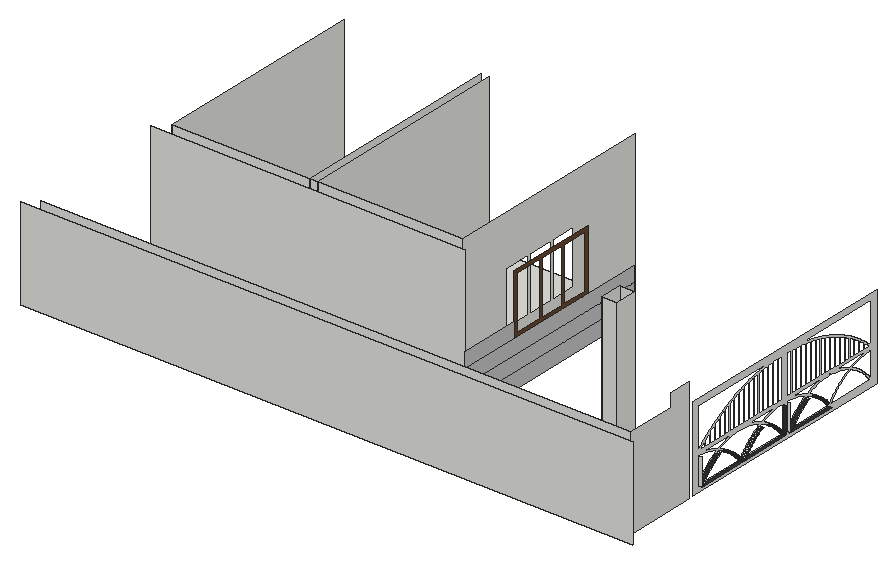
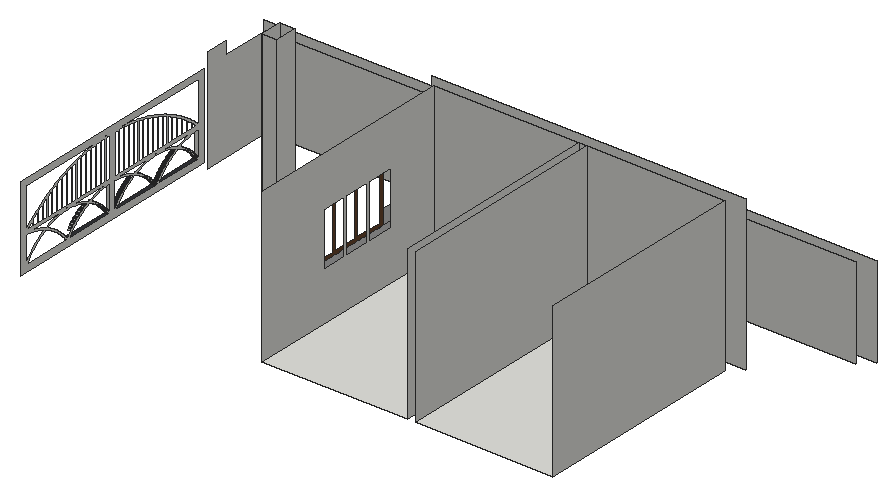
# SketchUp Ruby script. Lengths in inches.
U = 1.inch
M = Sketchup.active_model
def pt(a) = Geom::Point3d.new(a.map { |v| v * U })
def face(e, loops, mat)
  f = e.add_face(loops[0].map { |a| pt(a) })
  loops[1..].each { |l| e.add_face(l.map { |a| pt(a) }).erase! }
  f.material = f.back_material = mat if mat
  f
end
# faces: each face lists its corners as indices into pts; further lists are holes
def faces(e, pts, list, mat = nil) = list.each { |f| face(e, (f[0].is_a?(Array) ? f : [f]).map { |l| l.map { |i| pts[i] } }, mat) }
# xy, xz, yz: faces in a plane at the given z, y or x. An outline is a flat list of corners, or four numbers for a rectangle; further outlines are holes
def ring(l) = l.size == 4 ? [[l[0], l[1]], [l[2], l[1]], [l[2], l[3]], [l[0], l[3]]] : l.each_slice(2).to_a
def flat(e, list, mat, &to3) = list.each { |f| face(e, (f[0].is_a?(Array) ? f : [f]).map { |l| ring(l).map { |u, v| to3.(u, v) } }, mat) }
def xy(e, z, list, mat = nil) = flat(e, list, mat) { |x, y| [x, y, z] }
def xz(e, y, list, mat = nil) = flat(e, list, mat) { |x, z| [x, y, z] }
def yz(e, x, list, mat = nil) = flat(e, list, mat) { |y, z| [x, y, z] }
def lines(e, pts, list) = list.each { |a, b| e.add_line(pt(pts[a]), pt(pts[b])) }
# prism: a flat outline (further loops are holes) pulled along v
def prism(e, loops, v, mat = nil)
  f = face(e, loops, mat); d = Geom::Vector3d.new(v.map { |x| x * U })
  f.pushpull(f.normal.samedirection?(d) ? d.length : -d.length)
end
def box(e, o, s, mat = nil) = prism(e, [[o, [o[0] + s[0], o[1], o[2]], [o[0] + s[0], o[1] + s[1], o[2]], [o[0], o[1] + s[1], o[2]]]], [0, 0, s[2]], mat)
def at(x, y, z, deg = 0) = Geom::Transformation.translation(pt([x, y, z])) * Geom::Transformation.rotation(ORIGIN, Z_AXIS, deg.degrees)
def axes(o, x, y, z) = Geom::Transformation.new([*x, 0, *y, 0, *z, 0, *pt(o).to_a, 1])
def part(name) = M.definitions.add(name)
# library, detail: a bought-in or finely detailed component or shape, given as its bounding box
def library(name, o, s) = part(name).tap { |d| box(d.entities, o, s) }
def detail(e, o, s) = box(e.add_group.entities, o, s)
def put(e, d, t, mat = nil) = e.add_instance(d, t).tap { |i| i.material = mat if mat }
def group(e, t, mat = nil) = e.add_group.tap { |g| g.transformation = t; g.material = mat if mat }.entities
root = M.entities
M.materials.add("M02_Ash_Whisper").color = [196, 196, 196]
M.materials.add("ThomThom - Buttons1").color = [48, 49, 53]
M.materials.add("Wood_Veneer_15_1K").color = [103, 69, 45]
xy(root,24,[[66,66,174,234],[180,66,294,234]])
xy(root,32,[[474,72.225,477,111.313],[474,113.367,477,152.836],[474,159.225,477,198.633]],"ThomThom - Buttons1")
xz(root,0,[[0,24,480,96]])
xz(root,9,[[9,24,471,96]])
xz(root,57,[[57,24,303,144]])
xz(root,63,[[405,24,417,144]])
xz(root,66,[[66,24,174,144],[174,24,180,144],[180,24,294,144]])
xz(root,71,[[474,32,477,53.015]])
xz(root,81,[[405,24,417,144]])
xz(root,154,[[474,32,477,53.014]],"ThomThom - Buttons1")
xz(root,158,[[474,32,477,53.014]])
yz(root,66,[[66,24,234,144]])
yz(root,174,[[66,24,234,144]])
yz(root,180,[[66,24,234,144]])
yz(root,294,[[[66,24,234,144],[108,63,130,105],[132.007,62.883,152,105],[154.007,62.883,174,105]]])
yz(root,303,[[57,24,222,36],[57,36,222,48],[57,48,222,60],[57,60,105,72]],"M02_Ash_Whisper")
yz(root,303,[[[105,60,177,108],[132.007,62.883,132.007,104.883,130,105,130,63,108,63,108,105,130,105,132.007,104.883,152,105,154.007,104.883,174,105,174,63,154.007,62.883,154.007,104.883,152,105,152,63]]],"Wood_Veneer_15_1K")
yz(root,405,[[63,24,81,144]])
yz(root,417,[[63,24,81,144]])
yz(root,471,[[9,24,9,96,48,96,48,106,66,106,66,24]])
yz(root,474,[[[66,27,246,93],[241,56,241,88,161.003,88,161.646,87.994,163.468,87.949,165.29,87.877,167.11,87.776,168.929,87.648,170.745,87.493,172.559,87.309,174.37,87.098,176.177,86.859,177.98,86.593,179.779,86.299,181.574,85.977,183.363,85.629,185.147,85.253,186.925,84.85,188.696,84.42,190.461,83.962,192.219,83.478,193.969,82.967,195.711,82.43,197.444,81.866,199.169,81.275,200.885,80.659,202.59,80.016,204.286,79.347,205.972,78.653,207.647,77.932,209.31,77.187,210.962,76.416,212.602,75.62,214.23,74.799,215.845,73.953,217.446,73.082,219.035,72.1875,220.609,71.269,222.17,70.326,223.715,69.36,225.246,68.37,226.762,67.356,228.262,66.32,229.745,65.261,231.213,64.18,232.664,63.076,234.098,61.95,235.514,60.802,236.913,59.633,238.294,58.443,239.656,57.232],[71,56,72.344,57.232,73.588,58.338,73.706,58.443,75.087,59.633,76.486,60.802,77.902,61.95,78.318,62.277,79.336,63.076,80.787,64.18,82.255,65.261,83.048,65.828,83.738,66.32,85.238,67.356,86.754,68.37,87.778,69.032,88.285,69.36,89.83,70.326,91.391,71.269,92.509,71.921,92.965,72.1875,94.554,73.082,96.155,73.953,97.239,74.52,97.77,74.799,99.398,75.62,101.038,76.416,101.969,76.85,102.69,77.187,104.353,77.932,106.028,78.653,106.699,78.929,107.714,79.347,109.41,80.016,111.115,80.659,111.429,80.771,112.831,81.275,114.556,81.866,116.159,82.388,116.289,82.43,118.031,82.967,119.781,83.478,120.889,83.783,121.539,83.962,123.304,84.42,125.075,84.85,125.619,84.973,126.853,85.253,128.637,85.629,130.349,85.962,130.426,85.977,132.221,86.299,134.02,86.593,135.08,86.749,135.823,86.859,137.63,87.098,139.441,87.309,141.255,87.493,143.071,87.648,144.89,87.776,146.71,87.877,148.532,87.949,150.354,87.994,150.997,88,71,88],[199.66,32.254,200.052,32.779,200.649,33.547,201.259,34.304,201.883,35.05,202.52,35.784,203.171,36.507,203.834,37.218,204.51,37.918,205.198,38.604,205.899,39.279,206.612,39.94,207.336,40.589,208.072,41.225,208.819,41.847,209.578,42.455,210.347,43.05,211.127,43.631,211.917,44.198,212.718,44.751,213.528,45.288,214.347,45.812,215.176,46.32,216.014,46.814,216.861,47.292,217.716,47.755,218.58,48.202,219.451,48.634,219.589,48.7,218.181,49.31,216.395,50.004,214.583,50.628,212.748,51.18,210.893,51.661,209.021,52.069,207.134,52.403,205.236,52.664,203.329,52.85,201.416,52.962,199.5,53,197.584,52.962,195.671,52.85,193.764,52.664,191.866,52.403,189.979,52.069,188.107,51.661,186.252,51.18,184.417,50.628,182.605,50.004,180.819,49.31,179.578,48.772,179.731,48.7,179.869,48.634,180.74,48.202,181.604,47.755,182.459,47.292,183.306,46.814,184.144,46.32,184.973,45.812,185.792,45.288,186.602,44.751,187.403,44.198,188.193,43.631,188.973,43.05,189.742,42.455,190.501,41.847,191.248,41.225,191.984,40.589,192.708,39.94,193.421,39.279,194.122,38.604,194.81,37.918,195.486,37.218,196.149,36.507,196.8,35.784,197.437,35.05,198.061,34.304,198.671,33.547,199.268,32.779],[112.34,32.254,112.732,32.779,113.329,33.547,113.939,34.304,114.563,35.05,115.2,35.784,115.851,36.507,116.514,37.218,117.19,37.918,117.878,38.604,118.579,39.279,119.292,39.94,120.016,40.589,120.752,41.225,121.499,41.847,122.258,42.455,123.027,43.05,123.807,43.631,124.597,44.198,125.398,44.751,126.208,45.288,127.027,45.812,127.856,46.32,128.694,46.814,129.541,47.292,130.396,47.755,131.26,48.202,132.131,48.634,132.269,48.7,132.422,48.772,131.181,49.31,129.395,50.004,127.583,50.628,125.748,51.18,123.893,51.661,122.021,52.069,120.134,52.403,118.236,52.664,116.329,52.85,114.416,52.962,112.5,53,110.584,52.962,108.671,52.85,106.764,52.664,104.866,52.403,102.979,52.069,101.107,51.661,99.252,51.18,97.417,50.628,95.605,50.004,93.819,49.31,92.411,48.7,92.549,48.634,93.42,48.202,94.284,47.755,95.139,47.292,95.986,46.814,96.824,46.32,97.653,45.812,98.472,45.288,99.282,44.751,100.083,44.198,100.873,43.631,101.653,43.05,102.422,42.455,103.181,41.847,103.928,41.225,104.664,40.589,105.388,39.94,106.101,39.279,106.802,38.604,107.49,37.918,108.166,37.218,108.829,36.507,109.48,35.784,110.117,35.05,110.741,34.304,111.351,33.547,111.948,32.779],[113.367,32,152.836,32,152.066,33.003,150.9,34.524,149.675,35.997,148.394,37.422,147.058,38.796,145.669,40.117,144.231,41.382,142.744,42.591,141.21,43.741,139.634,44.83,138.016,45.856,136.359,46.819,134.666,47.717,133.583,48.238,131.712,47.31,130.864,46.871,130.025,46.417,129.194,45.947,128.371,45.463,127.558,44.964,126.753,44.45,125.958,43.922,125.173,43.38,124.397,42.824,123.632,42.254,122.877,41.67,122.132,41.073,121.399,40.462,120.676,39.838,119.965,39.201,119.266,38.552,118.578,37.89,117.903,37.216,117.239,36.53,116.588,35.832,115.95,35.122,115.325,34.401,114.712,33.669],[159.225,32,198.633,32,197.288,33.669,196.675,34.401,196.05,35.122,195.412,35.832,194.761,36.53,194.097,37.216,193.422,37.89,192.734,38.552,192.035,39.201,191.324,39.838,190.601,40.462,189.868,41.073,189.123,41.67,188.368,42.254,187.603,42.824,186.827,43.38,186.042,43.922,185.247,44.45,184.442,44.964,183.629,45.463,182.806,45.947,181.975,46.417,181.136,46.871,180.288,47.31,178.417,48.238,177.334,47.717,175.641,46.819,173.984,45.856,172.366,44.83,170.79,43.741,169.256,42.591,167.769,41.382,166.331,40.117,164.942,38.796,163.606,37.422,162.325,35.997,161.1,34.524,159.934,33.003,159.932,33],[72.225,32,111.313,32,110.507,33,109.968,33.669,109.355,34.401,108.73,35.122,108.092,35.832,107.441,36.53,106.778,37.216,106.102,37.89,105.414,38.552,104.715,39.201,104.004,39.838,103.281,40.462,102.548,41.073,101.803,41.67,101.048,42.254,100.283,42.824,99.507,43.38,98.722,43.922,97.927,44.45,97.122,44.964,96.309,45.463,95.486,45.947,94.655,46.417,93.816,46.871,92.968,47.31,92.391,47.597,91.195,48.131,90.334,47.717,88.641,46.819,86.984,45.856,85.366,44.83,83.79,43.741,82.256,42.591,80.769,41.382,79.331,40.117,77.942,38.796,76.606,37.422,75.325,35.997,74.1,34.524,72.934,33.003],[200.687,32,239.775,32,239.066,33.003,237.9,34.524,236.675,35.997,235.394,37.422,234.058,38.796,232.669,40.117,231.231,41.382,229.744,42.591,228.21,43.741,226.634,44.83,225.016,45.856,223.359,46.819,221.666,47.717,220.805,48.131,219.609,47.597,219.032,47.31,218.184,46.871,217.345,46.417,216.514,45.947,215.691,45.463,214.878,44.964,214.073,44.45,213.278,43.922,212.493,43.38,211.717,42.824,210.952,42.254,210.197,41.67,209.452,41.073,208.719,40.462,207.996,39.838,207.285,39.201,206.586,38.552,205.898,37.89,205.222,37.216,204.559,36.53,203.908,35.832,203.27,35.122,202.645,34.401,202.032,33.669,201.493,33],[154,32,154,53.014,152.764,52.957,151.811,52.896,150.86,52.818,149.91,52.722,148.962,52.61,148.017,52.481,147.074,52.334,146.133,52.171,145.196,51.991,144.262,51.793,143.332,51.58,142.406,51.349,141.484,51.102,140.567,50.838,139.654,50.558,138.747,50.261,137.845,49.948,136.949,49.619,136.06,49.274,134.719,48.801,135.117,48.609,136.845,47.694,138.535,46.711,140.186,45.664,141.795,44.552,143.359,43.379,144.876,42.146,146.345,40.855,147.761,39.507,149.124,38.105,150.432,36.652,151.681,35.148,152.871,33.597],[158,32,159.129,33.597,160.319,35.148,161.568,36.652,162.876,38.105,164.239,39.507,165.655,40.855,167.124,42.146,168.641,43.379,170.205,44.552,171.814,45.664,173.465,46.711,175.155,47.694,176.883,48.609,177.281,48.801,175.94,49.274,175.051,49.619,174.155,49.948,173.253,50.261,172.346,50.558,171.433,50.838,170.516,51.102,169.594,51.349,168.668,51.58,167.738,51.793,166.804,51.991,165.867,52.171,164.926,52.334,163.983,52.481,163.038,52.61,162.09,52.722,161.14,52.818,160.189,52.896,159.236,52.957,158,53.014],[241,32,241,53.015,240,52.951,239.131,52.896,238.18,52.818,237.23,52.722,236.282,52.61,235.337,52.481,234.394,52.334,233.453,52.171,232.516,51.991,231.582,51.793,230.652,51.58,229.726,51.349,228.804,51.102,227.887,50.838,226.974,50.558,226.067,50.261,225.165,49.948,224.269,49.619,223.38,49.274,223.165,49.186,222.001,48.665,222.117,48.609,223.845,47.694,225.535,46.711,227.186,45.664,228.795,44.552,230.359,43.379,231.876,42.146,233.345,40.855,234.761,39.507,236.124,38.105,237.432,36.652,238.681,35.148,239.871,33.597],[71,32,72.129,33.597,73.319,35.148,74.568,36.652,75.876,38.105,77.239,39.507,78.655,40.855,80.124,42.146,81.641,43.379,83.205,44.552,84.814,45.664,86.465,46.711,88.155,47.694,89.883,48.609,89.999,48.665,88.835,49.186,88.62,49.274,87.731,49.619,86.835,49.948,85.933,50.261,85.026,50.558,84.113,50.838,83.196,51.102,82.274,51.349,81.348,51.58,80.418,51.793,79.484,51.991,78.547,52.171,77.606,52.334,76.663,52.481,75.718,52.61,74.77,52.722,73.82,52.818,72.869,52.896,72,52.951,71,53.015],[149.37,56.1,153.9,56.1,153.9,86.9,151.002,86.9,150.373,86.894,149.37,86.87],[158.1,56.1,162.63,56.1,162.63,86.87,161.627,86.894,160.998,86.9,158.1,86.9],[144.64,56.1,149.17,56.1,149.17,86.865,148.567,86.85,146.762,86.778,144.959,86.679,144.64,86.656],[162.83,56.1,167.36,56.1,167.36,86.656,167.041,86.679,165.238,86.778,163.433,86.85,162.83,86.865],[139.91,56.1,144.44,56.1,144.44,86.642,143.157,86.552,141.357,86.397,139.91,86.251],[167.56,56.1,172.09,56.1,172.09,86.251,170.643,86.397,168.843,86.552,167.56,86.642],[135.18,56.1,139.71,56.1,139.71,86.231,139.56,86.215,137.766,86.006,135.976,85.77,135.18,85.652],[172.29,56.1,176.82,56.1,176.82,85.652,176.024,85.77,174.234,86.006,172.44,86.215,172.29,86.231],[130.449,56.1,134.98,56.1,134.98,85.622,134.189,85.506,132.406,85.214,130.628,84.896,130.449,84.861],[177.02,56.1,181.551,56.1,181.551,84.861,181.372,84.896,179.594,85.214,177.811,85.506,177.02,85.622],[125.719,56.1,130.249,56.1,130.249,84.822,128.855,84.551,127.088,84.178,125.719,83.868],[181.751,56.1,186.281,56.1,186.281,83.868,184.912,84.178,183.145,84.551,181.751,84.822],[186.481,56.1,191.011,56.1,191.011,82.67,190.177,82.9,188.429,83.353,186.674,83.779,186.481,83.823],[120.989,56.1,125.519,56.1,125.519,83.823,125.326,83.779,123.571,83.353,121.823,82.9,120.989,82.67],[116.259,56.1,120.789,56.1,120.789,82.615,120.081,82.42,118.348,81.914,116.622,81.381,116.259,81.263],[191.211,56.1,195.741,56.1,195.741,81.263,195.378,81.381,193.652,81.914,191.919,82.42,191.211,82.615],[111.529,56.1,116.059,56.1,116.059,81.198,114.904,80.822,113.195,80.237,111.529,79.639],[195.941,56.1,200.471,56.1,200.471,79.639,198.805,80.237,197.096,80.822,195.941,81.198],[106.799,56.1,111.329,56.1,111.329,79.564,109.805,78.99,108.125,78.327,106.799,77.781],[200.671,56.1,205.201,56.1,205.201,77.781,203.875,78.327,202.195,78.99,200.671,79.564],[205.401,56.1,209.931,56.1,209.931,75.683,208.853,76.186,207.204,76.925,205.545,77.639,205.401,77.698],[102.069,56.1,106.599,56.1,106.599,77.698,106.455,77.639,104.796,76.925,103.147,76.186,102.069,75.683],[97.339,56.1,101.869,56.1,101.869,75.59,101.511,75.423,99.886,74.634,98.273,73.82,97.339,73.331],[210.131,56.1,214.661,56.1,214.661,73.331,213.727,73.82,212.114,74.634,210.489,75.423,210.131,75.59],[92.609,56.1,97.139,56.1,97.139,73.226,96.673,72.982,95.086,72.12,93.512,71.233,92.609,70.706],[214.861,56.1,219.391,56.1,219.391,70.706,218.488,71.233,216.914,72.12,215.327,72.982,214.861,73.226],[220.779,49.253,221.216,49.45,222.109,49.835,223.01,50.203,223.916,50.554,224.829,50.89,225.748,51.209,226.672,51.511,227.601,51.796,228.536,52.065,229.475,52.317,230.419,52.552,231.367,52.77,232.318,52.971,233.273,53.155,234.231,53.321,235.192,53.47,236.156,53.602,237.121,53.716,238.089,53.814,239.058,53.893,240.029,53.955,241,54,199.5,54,201.455,53.962,203.407,53.848,205.353,53.657,207.29,53.391,209.215,53.05,211.125,52.634,213.018,52.143,214.89,51.58,216.739,50.943,218.562,50.236,220.355,49.457],[91.221,49.253,91.645,49.457,93.438,50.236,95.261,50.943,97.11,51.58,98.982,52.143,100.875,52.634,102.785,53.05,104.71,53.391,106.647,53.657,108.593,53.848,110.545,53.962,112.5,54,71,54,71.971,53.955,72.942,53.893,73.911,53.814,74.879,53.716,75.844,53.602,76.808,53.47,77.769,53.321,78.727,53.155,79.682,52.971,80.633,52.77,81.581,52.552,82.525,52.317,83.464,52.065,84.399,51.796,85.328,51.511,86.252,51.209,87.171,50.89,88.084,50.554,88.99,50.203,89.891,49.835,90.784,49.45],[178.376,49.328,178.645,49.457,180.438,50.236,182.261,50.943,184.11,51.58,185.982,52.143,187.875,52.634,189.785,53.05,191.71,53.391,193.647,53.657,195.593,53.848,197.545,53.962,199.5,54,158.32,54,159.291,53.955,160.262,53.893,161.231,53.814,162.199,53.716,163.164,53.602,164.128,53.47,165.089,53.321,166.047,53.155,167.002,52.971,167.953,52.77,168.901,52.552,169.845,52.317,170.784,52.065,171.718,51.796,172.648,51.511,173.572,51.209,174.491,50.89,175.404,50.554,176.31,50.203,177.211,49.835,178.104,49.45],[133.624,49.328,133.896,49.45,134.789,49.835,135.69,50.203,136.596,50.554,137.509,50.89,138.428,51.209,139.352,51.511,140.282,51.796,141.216,52.065,142.155,52.317,143.099,52.552,144.047,52.77,144.998,52.971,145.953,53.155,146.911,53.321,147.872,53.47,148.836,53.602,149.801,53.716,150.769,53.814,151.738,53.893,152.709,53.955,153.68,54,112.5,54,114.455,53.962,116.407,53.848,118.353,53.657,120.29,53.391,122.215,53.05,124.125,52.634,126.018,52.143,127.89,51.58,129.739,50.943,131.562,50.236,133.355,49.457],[87.878,56.1,92.409,56.1,92.409,70.589,91.952,70.323,90.406,69.389,88.875,68.431,87.878,67.787],[219.591,56.1,224.122,56.1,224.122,67.787,223.125,68.431,221.594,69.389,220.048,70.323,219.591,70.589],[83.148,56.1,87.678,56.1,87.678,67.658,87.358,67.45,85.857,66.447,84.371,65.42,83.148,64.548],[224.322,56.1,228.852,56.1,228.852,64.548,227.629,65.42,226.143,66.447,224.642,67.45,224.322,67.658],[229.052,56.1,233.582,56.1,233.582,60.952,233.412,61.09,231.991,62.205,230.554,63.299,229.1,64.371,229.052,64.405],[78.418,56.1,82.948,56.1,82.948,64.405,82.9,64.371,81.446,63.299,80.009,62.205,78.588,61.09,78.418,60.952],[73.688,56.1,78.218,56.1,78.218,60.79,77.185,59.953,75.799,58.795,74.431,57.615,73.688,56.955],[233.782,56.1,238.312,56.1,238.312,56.955,237.569,57.615,236.201,58.795,234.815,59.953,233.782,60.79]]])
p = [[477,71,32],[477,72.129,33.597],[474,72.129,33.597],[474,71,32],[477,72.934,33.003],[477,72.225,32],
  [474,72.225,32],[474,72.934,33.003],[477,111.313,32],[477,110.507,33],[474,110.507,33],[474,111.313,32],
  [477,114.712,33.669],[477,113.367,32],[474,113.367,32],[474,114.712,33.669],[477,152.836,32],[477,152.066,33.003],
  [474,152.066,33.003],[474,152.836,32],[477,152.871,33.597],[477,154,32],[474,154,32],[474,152.871,33.597],
  [477,158,32],[477,159.129,33.597],[474,159.129,33.597],[474,158,32],[477,159.932,33],[477,159.225,32],
  [474,159.225,32],[474,159.932,33],[477,111.948,32.779],[477,112.34,32.254],[474,112.34,32.254],[474,111.948,32.779],
  [477,112.732,32.779],[474,112.732,32.779],[477,111.351,33.547],[474,111.351,33.547],[477,113.329,33.547],[474,113.329,33.547],
  [477,74.1,34.524],[474,74.1,34.524],[477,109.968,33.669],[474,109.968,33.669],[477,150.9,34.524],[474,150.9,34.524],
  [477,159.934,33.003],[474,159.934,33.003],[477,161.1,34.524],[474,161.1,34.524],[477,110.741,34.304],[474,110.741,34.304],
  [477,113.939,34.304],[474,113.939,34.304],[477,73.319,35.148],[474,73.319,35.148],[477,151.681,35.148],[474,151.681,35.148],
  [477,160.319,35.148],[474,160.319,35.148],[477,109.355,34.401],[474,109.355,34.401],[477,115.325,34.401],[474,115.325,34.401],
  [477,110.117,35.05],[474,110.117,35.05],[477,114.563,35.05],[474,114.563,35.05],[477,108.73,35.122],[474,108.73,35.122],
  [477,115.95,35.122],[474,115.95,35.122],[477,75.325,35.997],[474,75.325,35.997],[477,149.675,35.997],[474,149.675,35.997],
  [477,162.325,35.997],[474,162.325,35.997],[477,109.48,35.784],[474,109.48,35.784],[477,115.2,35.784],[474,115.2,35.784],
  [477,74.568,36.652],[474,74.568,36.652],[477,108.092,35.832],[474,108.092,35.832],[477,116.588,35.832],[474,116.588,35.832],
  [477,150.432,36.652],[474,150.432,36.652],[477,161.568,36.652],[474,161.568,36.652],[477,107.441,36.53],[474,107.441,36.53],
  [477,108.829,36.507],[474,108.829,36.507],[477,115.851,36.507],[474,115.851,36.507],[477,117.239,36.53],[474,117.239,36.53],
  [477,195.412,35.832],[477,194.761,36.53],[474,194.761,36.53],[474,195.412,35.832],[477,76.606,37.422],[474,76.606,37.422],
  [477,148.394,37.422],[474,148.394,37.422],[477,163.606,37.422],[474,163.606,37.422],[477,106.778,37.216],[474,106.778,37.216],
  [477,108.166,37.218],[474,108.166,37.218],[477,116.514,37.218],[474,116.514,37.218],[477,117.903,37.216],[474,117.903,37.216],
  [477,194.097,37.216],[474,194.097,37.216],[477,75.876,38.105],[474,75.876,38.105],[477,149.124,38.105],[474,149.124,38.105],
  [477,162.876,38.105],[474,162.876,38.105],[477,106.102,37.89],[474,106.102,37.89],[477,107.49,37.918],[474,107.49,37.918],
  [477,117.19,37.918],[474,117.19,37.918],[477,118.578,37.89],[474,118.578,37.89],[477,193.422,37.89],[474,193.422,37.89],
  [477,77.942,38.796],[474,77.942,38.796],[477,147.058,38.796],[474,147.058,38.796],[477,164.942,38.796],[474,164.942,38.796],
  [477,105.414,38.552],[474,105.414,38.552],[477,106.802,38.604],[474,106.802,38.604],[477,117.878,38.604],[474,117.878,38.604],
  [477,119.266,38.552],[474,119.266,38.552],[477,192.734,38.552],[474,192.734,38.552],[477,194.122,38.604],[477,194.81,37.918],
  [474,194.81,37.918],[474,194.122,38.604],[477,77.239,39.507],[474,77.239,39.507],[477,147.761,39.507],[474,147.761,39.507],
  [477,164.239,39.507],[474,164.239,39.507],[477,104.715,39.201],[474,104.715,39.201],[477,106.101,39.279],[474,106.101,39.279],
  [477,118.579,39.279],[474,118.579,39.279],[477,119.965,39.201],[474,119.965,39.201],[477,192.035,39.201],[474,192.035,39.201],
  [477,193.421,39.279],[474,193.421,39.279],[477,79.331,40.117],[474,79.331,40.117],[477,145.669,40.117],[474,145.669,40.117],
  [477,166.331,40.117],[474,166.331,40.117],[477,104.004,39.838],[474,104.004,39.838],[477,120.676,39.838],[474,120.676,39.838],
  [477,191.324,39.838],[474,191.324,39.838],[477,105.388,39.94],[474,105.388,39.94],[477,119.292,39.94],[474,119.292,39.94],
  [477,192.708,39.94],[474,192.708,39.94],[477,78.655,40.855],[474,78.655,40.855],[477,146.345,40.855],[474,146.345,40.855],
  [477,165.655,40.855],[474,165.655,40.855],[477,103.281,40.462],[474,103.281,40.462],[477,121.399,40.462],[474,121.399,40.462],
  [477,190.601,40.462],[474,190.601,40.462],[477,104.664,40.589],[474,104.664,40.589],[477,120.016,40.589],[474,120.016,40.589],
  [477,191.984,40.589],[474,191.984,40.589],[477,80.769,41.382],[474,80.769,41.382],[477,144.231,41.382],[474,144.231,41.382],
  [477,167.769,41.382],[474,167.769,41.382],[477,102.548,41.073],[474,102.548,41.073],[477,122.132,41.073],[474,122.132,41.073],
  [477,189.868,41.073],[474,189.868,41.073],[477,103.928,41.225],[474,103.928,41.225],[477,120.752,41.225],[474,120.752,41.225],
  [477,191.248,41.225],[474,191.248,41.225],[477,80.124,42.146],[474,80.124,42.146],[477,144.876,42.146],[474,144.876,42.146],
  [477,167.124,42.146],[474,167.124,42.146],[477,101.803,41.67],[474,101.803,41.67],[477,122.877,41.67],[474,122.877,41.67],
  [477,189.123,41.67],[474,189.123,41.67],[477,103.181,41.847],[474,103.181,41.847],[477,121.499,41.847],[474,121.499,41.847],
  [477,190.501,41.847],[474,190.501,41.847],[477,82.256,42.591],[474,82.256,42.591],[477,142.744,42.591],[474,142.744,42.591],
  [477,169.256,42.591],[474,169.256,42.591],[477,101.048,42.254],[474,101.048,42.254],[477,123.632,42.254],[474,123.632,42.254],
  [477,188.368,42.254],[474,188.368,42.254],[477,102.422,42.455],[474,102.422,42.455],[477,122.258,42.455],[474,122.258,42.455],
  [477,189.742,42.455],[474,189.742,42.455],[477,81.641,43.379],[474,81.641,43.379],[477,143.359,43.379],[474,143.359,43.379],
  [477,168.641,43.379],[474,168.641,43.379],[477,100.283,42.824],[474,100.283,42.824],[477,124.397,42.824],[474,124.397,42.824],
  [477,187.603,42.824],[474,187.603,42.824],[477,101.653,43.05],[474,101.653,43.05],[477,123.027,43.05],[474,123.027,43.05],
  [477,188.973,43.05],[474,188.973,43.05],[477,83.79,43.741],[474,83.79,43.741],[477,141.21,43.741],[474,141.21,43.741],
  [477,170.79,43.741],[474,170.79,43.741],[477,99.507,43.38],[474,99.507,43.38],[477,125.173,43.38],[474,125.173,43.38],
  [477,186.827,43.38],[474,186.827,43.38],[477,100.873,43.631],[474,100.873,43.631],[477,123.807,43.631],[474,123.807,43.631],
  [477,188.193,43.631],[474,188.193,43.631],[477,83.205,44.552],[474,83.205,44.552],[477,98.722,43.922],[474,98.722,43.922],
  [477,125.958,43.922],[474,125.958,43.922],[477,141.795,44.552],[474,141.795,44.552],[477,170.205,44.552],[474,170.205,44.552],
  [477,186.042,43.922],[474,186.042,43.922],[477,100.083,44.198],[474,100.083,44.198],[477,124.597,44.198],[474,124.597,44.198],
  [477,187.403,44.198],[474,187.403,44.198],[477,85.366,44.83],[474,85.366,44.83],[477,139.634,44.83],[474,139.634,44.83],
  [477,172.366,44.83],[474,172.366,44.83],[477,97.927,44.45],[474,97.927,44.45],[477,126.753,44.45],[474,126.753,44.45],
  [477,185.247,44.45],[474,185.247,44.45],[477,99.282,44.751],[474,99.282,44.751],[477,125.398,44.751],[474,125.398,44.751],
  [477,186.602,44.751],[474,186.602,44.751],[477,97.122,44.964],[474,97.122,44.964],[477,127.558,44.964],[474,127.558,44.964],
  [477,184.442,44.964],[474,184.442,44.964],[477,84.814,45.664],[474,84.814,45.664],[477,140.186,45.664],[474,140.186,45.664],
  [477,171.814,45.664],[474,171.814,45.664],[477,86.984,45.856],[474,86.984,45.856],[477,98.472,45.288],[474,98.472,45.288],
  [477,126.208,45.288],[474,126.208,45.288],[477,138.016,45.856],[474,138.016,45.856],[477,173.984,45.856],[474,173.984,45.856],
  [477,185.792,45.288],[474,185.792,45.288],[477,96.309,45.463],[474,96.309,45.463],[477,128.371,45.463],[474,128.371,45.463],
  [477,183.629,45.463],[474,183.629,45.463],[477,97.653,45.812],[474,97.653,45.812],[477,127.027,45.812],[474,127.027,45.812],
  [477,184.973,45.812],[474,184.973,45.812],[477,95.486,45.947],[474,95.486,45.947],[477,129.194,45.947],[474,129.194,45.947],
  [477,182.806,45.947],[474,182.806,45.947],[477,86.465,46.711],[474,86.465,46.711],[477,138.535,46.711],[474,138.535,46.711],
  [477,173.465,46.711],[474,173.465,46.711],[477,96.824,46.32],[474,96.824,46.32],[477,127.856,46.32],[474,127.856,46.32],
  [477,184.144,46.32],[474,184.144,46.32],[477,88.641,46.819],[474,88.641,46.819],[477,94.655,46.417],[474,94.655,46.417],
  [477,130.025,46.417],[474,130.025,46.417],[477,136.359,46.819],[474,136.359,46.819],[477,175.641,46.819],[474,175.641,46.819],
  [477,181.975,46.417],[474,181.975,46.417],[477,95.986,46.814],[474,95.986,46.814],[477,128.694,46.814],[474,128.694,46.814],
  [477,183.306,46.814],[474,183.306,46.814],[477,93.816,46.871],[474,93.816,46.871],[477,130.864,46.871],[474,130.864,46.871],
  [477,181.136,46.871],[474,181.136,46.871],[477,88.155,47.694],[474,88.155,47.694],[477,136.845,47.694],[474,136.845,47.694],
  [477,175.155,47.694],[474,175.155,47.694],[477,90.334,47.717],[474,90.334,47.717],[477,95.139,47.292],[474,95.139,47.292],
  [477,129.541,47.292],[474,129.541,47.292],[477,134.666,47.717],[474,134.666,47.717],[477,177.334,47.717],[474,177.334,47.717],
  [477,182.459,47.292],[474,182.459,47.292],[477,92.968,47.31],[474,92.968,47.31],[477,131.712,47.31],[474,131.712,47.31],
  [477,180.288,47.31],[474,180.288,47.31],[477,94.284,47.755],[474,94.284,47.755],[477,130.396,47.755],[474,130.396,47.755],
  [477,181.604,47.755],[474,181.604,47.755]]
faces(root,p,[[0,1,2,3],[20,21,22,23],[24,25,26,27],[32,33,34,35],[38,32,35,39],[52,38,39,53],[1,56,57,2],[58,20,23,59],
  [25,60,61,26],[66,52,53,67],[80,66,67,81],[56,84,85,57],[90,58,59,91],[60,92,93,61],[96,80,81,97],[114,96,97,115],
  [84,122,123,85],[124,90,91,125],[92,126,127,93],[130,114,115,131],[146,130,131,147],[122,158,159,123],[160,124,125,161],[126,162,163,127],
  [166,146,147,167],[188,166,167,189],[158,194,195,159],[196,160,161,197],[162,198,199,163],[206,188,189,207],[224,206,207,225],[194,230,231,195],
  [232,196,197,233],[198,234,235,199],[242,224,225,243],[260,242,243,261],[230,266,267,231],[268,232,233,269],[234,270,271,235],[278,260,261,279],
  [296,278,279,297],[266,302,303,267],[308,268,269,309],[270,310,311,271],[314,296,297,315],[332,314,315,333],[302,344,345,303],[346,308,309,347],
  [310,348,349,311],[352,332,333,353],[368,352,353,369],[344,380,381,345],[382,346,347,383],[348,384,385,349],[386,368,369,387],[404,386,387,405],
  [380,416,417,381],[418,382,383,419],[384,420,421,385],[424,404,405,425],[440,424,425,441]],"ThomThom - Buttons1")
faces(root,p,[[4,5,6,7],[8,9,10,11],[12,13,14,15],[16,17,18,19],[28,29,30,31],[33,36,37,34],[36,40,41,37],[42,4,7,43],
  [9,44,45,10],[17,46,47,18],[48,28,31,49],[50,48,49,51],[40,54,55,41],[44,62,63,45],[64,12,15,65],[54,68,69,55],
  [62,70,71,63],[72,64,65,73],[74,42,43,75],[46,76,77,47],[78,50,51,79],[68,82,83,69],[70,86,87,71],[88,72,73,89],
  [86,94,95,87],[82,98,99,83],[100,88,89,101],[102,103,104,105],[106,74,75,107],[76,108,109,77],[110,78,79,111],[94,112,113,95],
  [98,116,117,99],[118,100,101,119],[103,120,121,104],[112,128,129,113],[116,132,133,117],[134,118,119,135],[120,136,137,121],[138,106,107,139],
  [108,140,141,109],[142,110,111,143],[128,144,145,129],[132,148,149,133],[150,134,135,151],[136,152,153,137],[154,155,156,157],[144,164,165,145],
  [148,168,169,149],[170,150,151,171],[152,172,173,153],[174,154,157,175],[176,138,139,177],[140,178,179,141],[180,142,143,181],[164,182,183,165],
  [184,170,171,185],[172,186,187,173],[168,190,191,169],[192,174,175,193],[182,200,201,183],[202,184,185,203],[186,204,205,187],[190,208,209,191],
  [210,192,193,211],[212,176,177,213],[178,214,215,179],[216,180,181,217],[200,218,219,201],[220,202,203,221],[204,222,223,205],[208,226,227,209],
  [228,210,211,229],[218,236,237,219],[238,220,221,239],[222,240,241,223],[226,244,245,227],[246,228,229,247],[248,212,213,249],[214,250,251,215],
  [252,216,217,253],[236,254,255,237],[256,238,239,257],[240,258,259,241],[244,262,263,245],[264,246,247,265],[254,272,273,255],[274,256,257,275],
  [258,276,277,259],[262,280,281,263],[282,264,265,283],[284,248,249,285],[250,286,287,251],[288,252,253,289],[272,290,291,273],[292,274,275,293],
  [276,294,295,277],[280,298,299,281],[300,282,283,301],[290,304,305,291],[306,292,293,307],[294,312,313,295],[298,316,317,299],[318,300,301,319],
  [320,284,285,321],[286,322,323,287],[324,288,289,325],[304,326,327,305],[328,306,307,329],[312,330,331,313],[316,334,335,317],[336,318,319,337],
  [326,338,339,327],[340,328,329,341],[330,342,343,331],[350,320,321,351],[334,354,355,335],[322,356,357,323],[358,324,325,359],[360,336,337,361],
  [338,362,363,339],[364,340,341,365],[342,366,367,343],[354,370,371,355],[372,360,361,373],[362,374,375,363],[376,364,365,377],[366,378,379,367],
  [370,388,389,371],[390,372,373,391],[392,350,351,393],[374,394,395,375],[396,376,377,397],[356,398,399,357],[400,358,359,401],[378,402,403,379],
  [388,406,407,389],[408,390,391,409],[394,410,411,395],[412,396,397,413],[402,414,415,403],[422,392,393,423],[406,426,427,407],[398,428,429,399],
  [430,400,401,431],[432,408,409,433],[410,434,435,411],[436,412,413,437],[414,438,439,415],[426,442,443,427],[444,432,433,445]])
